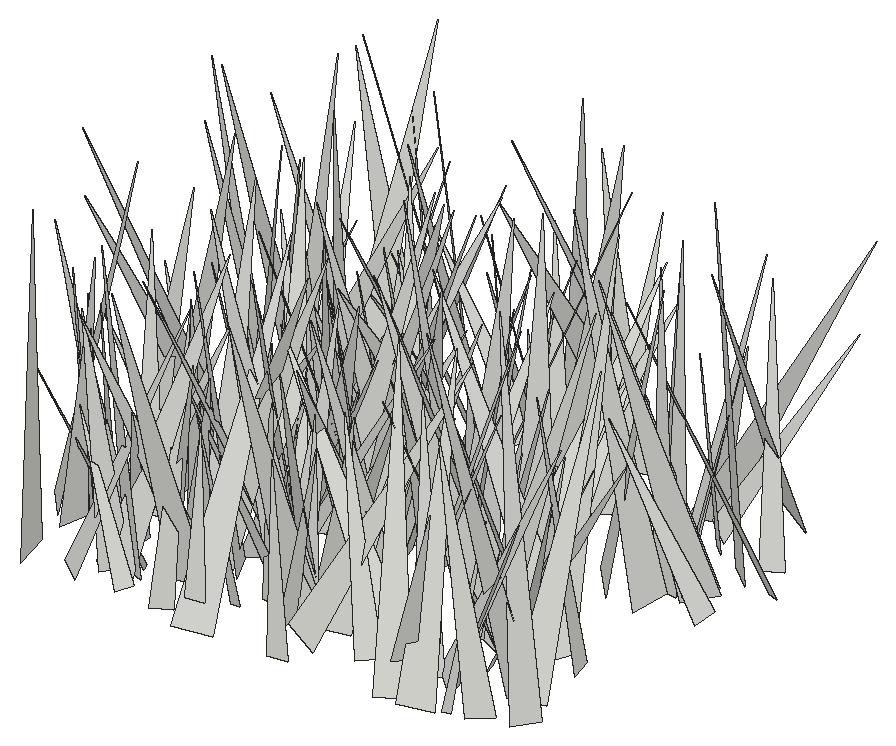
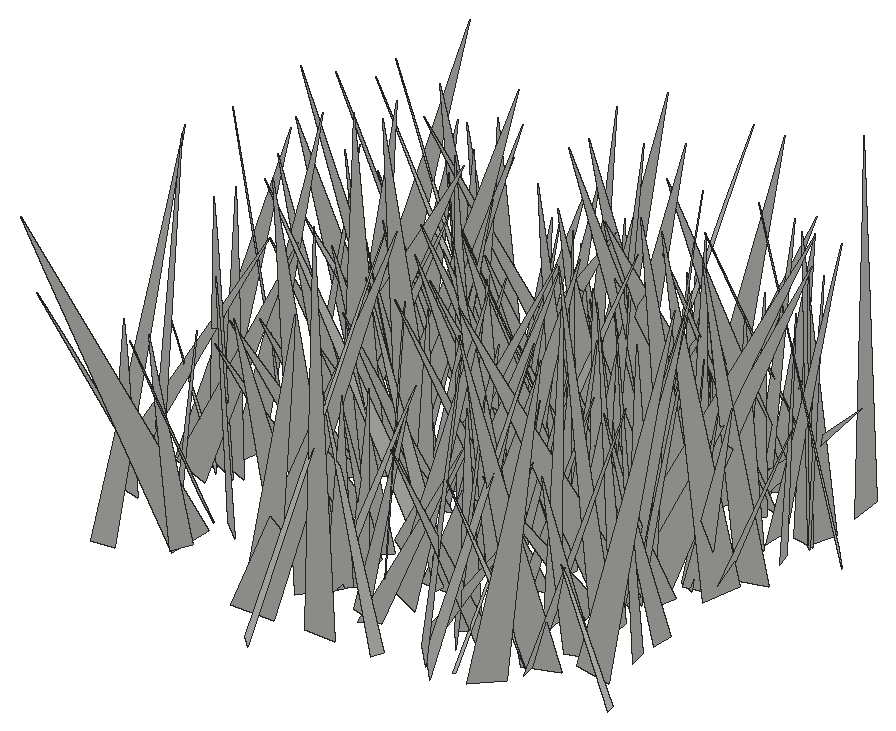
# SketchUp Ruby script. Lengths in inches.
U = 1.inch
M = Sketchup.active_model
def pt(a) = Geom::Point3d.new(a.map { |v| v * U })
def face(e, loops, mat)
  f = e.add_face(loops[0].map { |a| pt(a) })
  loops[1..].each { |l| e.add_face(l.map { |a| pt(a) }).erase! }
  f.material = f.back_material = mat if mat
  f
end
# faces: each face lists its corners as indices into pts; further lists are holes
def faces(e, pts, list, mat = nil) = list.each { |f| face(e, (f[0].is_a?(Array) ? f : [f]).map { |l| l.map { |i| pts[i] } }, mat) }
# xy, xz, yz: faces in a plane at the given z, y or x. An outline is a flat list of corners, or four numbers for a rectangle; further outlines are holes
def ring(l) = l.size == 4 ? [[l[0], l[1]], [l[2], l[1]], [l[2], l[3]], [l[0], l[3]]] : l.each_slice(2).to_a
def flat(e, list, mat, &to3) = list.each { |f| face(e, (f[0].is_a?(Array) ? f : [f]).map { |l| ring(l).map { |u, v| to3.(u, v) } }, mat) }
def xy(e, z, list, mat = nil) = flat(e, list, mat) { |x, y| [x, y, z] }
def xz(e, y, list, mat = nil) = flat(e, list, mat) { |x, z| [x, y, z] }
def yz(e, x, list, mat = nil) = flat(e, list, mat) { |y, z| [x, y, z] }
def lines(e, pts, list) = list.each { |a, b| e.add_line(pt(pts[a]), pt(pts[b])) }
# prism: a flat outline (further loops are holes) pulled along v
def prism(e, loops, v, mat = nil)
  f = face(e, loops, mat); d = Geom::Vector3d.new(v.map { |x| x * U })
  f.pushpull(f.normal.samedirection?(d) ? d.length : -d.length)
end
def box(e, o, s, mat = nil) = prism(e, [[o, [o[0] + s[0], o[1], o[2]], [o[0] + s[0], o[1] + s[1], o[2]], [o[0], o[1] + s[1], o[2]]]], [0, 0, s[2]], mat)
def at(x, y, z, deg = 0) = Geom::Transformation.translation(pt([x, y, z])) * Geom::Transformation.rotation(ORIGIN, Z_AXIS, deg.degrees)
def axes(o, x, y, z) = Geom::Transformation.new([*x, 0, *y, 0, *z, 0, *pt(o).to_a, 1])
def part(name) = M.definitions.add(name)
# library, detail: a bought-in or finely detailed component or shape, given as its bounding box
def library(name, o, s) = part(name).tap { |d| box(d.entities, o, s) }
def detail(e, o, s) = box(e.add_group.entities, o, s)
def put(e, d, t, mat = nil) = e.add_instance(d, t).tap { |i| i.material = mat if mat }
def group(e, t, mat = nil) = e.add_group.tap { |g| g.transformation = t; g.material = mat if mat }.entities
root = M.entities
c1 = part("fur_instance\#9")
p = [[0.8125,0,1.79],[0.67,-0.02,1.48],[0,-0.11,0],[0,0.11,0]]
faces(c1.entities,p,[[0,1,2,3]])
put(root,c1,axes([494.97,21.67,-21.86],[-0.42877,3.87256,1.55947],[4.17346,0.35848,0.25729],[-0.1042,-1.57711,3.88772]))
put(root,c1,axes([482.625,22.34,-21.86],[7.19679,1.10507,2.93039],[1.40985,-7.70082,-0.55845],[-2.79655,-1.03845,7.25969]))
put(root,c1,axes([499.85,22.83,-21.86],[2.67886,-4.09104,0.57639],[-4.11516,-2.58128,0.80469],[0.36641,0.91951,4.82342]))
put(root,c1,axes([490.95,21.67,-21.86],[-3.06481,2.41196,1.362],[2.48233,3.29293,-0.24563],[1.22908,-0.63618,3.89234]))
put(root,c1,axes([488.76,24.21,-21.86],[1.44091,-6.85532,1.40735],[-6.89305,-1.6385,-0.92385],[-1.20912,1.1714,6.94393]))
put(root,c1,axes([487.16,22.27,-21.86],[-3.33504,1.53851,0.16438],[1.54705,3.32218,0.29368],[0.02564,-0.33558,3.66104]))
put(root,c1,axes([485.94,23.24,-21.86],[3.52477,-3.78027,2.43443],[-3.94318,-4.08529,-0.63451],[-2.1606,1.28874,5.1295]))
put(root,c1,axes([493.65,24.95,-21.86],[2.47706,-6.70826,1.39737],[-6.69174,-2.68793,-1.04158],[-1.47445,0.92925,7.07472]))
put(root,c1,axes([503.74,22.87,-21.86],[-2.10663,5.00928,1.58804],[5.23429,1.84857,1.1125],[-0.46582,-1.88217,5.31913]))
put(root,c1,axes([488.68,25.03,-21.86],[1.14957,-5.99203,1.40359],[-5.68779,-1.57972,-2.08556],[-2.35023,0.89221,5.73379]))
put(root,c1,axes([484.65,22.14,-21.86],[3.5807,5.01538,0.32607],[5.01642,-3.54168,-0.61141],[0.30977,-0.61982,6.13202]))
put(root,c1,axes([493.22,25.93,-21.86],[-2.08812,-6.42397,1.05341],[-6.15561,2.30841,1.87538],[2.11792,0.37569,6.48927]))
put(root,c1,axes([501.36,21.95,-21.86],[-1.91608,6.79372,1.10059],[6.8739,1.94553,-0.04218],[0.33984,-1.04766,7.05863]))
put(root,c1,axes([500.21,22.02,-21.86],[-2.69969,6.39263,0.77147],[6.43614,2.65406,0.5304],[-0.19237,-0.91623,6.91901]))
put(root,c1,axes([485.48,25.29,-21.86],[4.01305,-1.4697,0.35123],[-1.33059,-3.90931,-1.15533],[-0.71618,-0.97223,4.11458]))
put(root,c1,axes([486.75,23.35,-21.86],[-3.5063,-5.04513,2.56803],[-5.65565,3.25438,-1.32851],[0.24851,2.88062,5.99854]))
put(root,c1,axes([493.62,23.95,-21.86],[3.83893,-0.81047,1.08867],[-0.8917,-3.9684,0.19003],[-1.0232,0.41758,3.91895]))
put(root,c1,axes([501.65,23.85,-21.86],[4.10602,0.97464,0.35289],[0.9844,-4.11806,-0.08026],[-0.32469,-0.15985,4.21935]))
put(root,c1,axes([504.2,24.85,-21.86],[-1.47229,-7.46087,2.3597],[-7.72207,0.99683,-1.66627],[-1.2659,2.59656,7.41996]))
put(root,c1,axes([491.17,23.9,-21.86],[0.98464,3.25356,1.70885],[3.23357,-1.6077,1.19779],[-1.74639,-1.14237,3.18127]))
put(root,c1,axes([498.42,24.57,-21.86],[5.98331,3.57339,0.75673],[3.63565,-5.68637,-1.89446],[0.35186,-2.00943,6.70672]))
put(root,c1,axes([502.5,22.4,-21.86],[1.53322,3.39,0.04746],[3.12816,-1.43461,1.41479],[-1.30727,0.54307,3.44111]))
put(root,c1,axes([489.17,21.97,-21.86],[-5.33411,1.7362,0.45715],[1.45522,5.02033,-2.08679],[1.05153,1.85957,5.20696]))
put(root,c1,axes([501.01,24.16,-21.86],[3.86219,5.07234,0.99731],[5.04282,-3.42294,-2.11973],[1.1372,-2.04809,6.01264]))
put(root,c1,axes([497.7,23.73,-21.86],[-2.79772,3.91125,0.86225],[4.00509,2.73873,0.57209],[0.02536,-1.03446,4.77471]))
put(root,c1,axes([486,23.1,-21.86],[-0.17372,7.00266,1.70424],[6.95108,0.61311,-1.81067],[1.90374,-1.5996,6.76675]))
put(root,c1,axes([486.73,24.05,-21.86],[-3.03964,-3.22245,0.08473],[-2.53096,2.3136,-2.80576],[-1.9964,1.97328,3.42802]))
put(root,c1,axes([482.43,25.15,-21.86],[5.9168,-1.45412,1.7202],[-1.44139,-6.15974,-0.24915],[-1.73089,0.15879,6.08776]))
put(root,c1,axes([486.95,25.27,-21.86],[4.77554,-0.30271,1.03368],[-0.19329,-4.86277,-0.53104],[-1.0596,-0.47722,4.75556]))
put(root,c1,axes([500.22,24.13,-21.86],[2.13883,-4.28297,3.06723],[-5.00629,-2.68295,-0.2554],[-1.63976,2.60467,4.7805]))
put(root,c1,axes([500.2,24.65,-21.86],[3.13012,3.09581,1.75638],[3.35561,-3.34662,-0.08138],[-1.18695,-1.29717,4.40172]))
put(root,c1,axes([489.71,28.34,-21.86],[-5.6893,-5.57398,0.54513],[-5.22917,5.56506,2.3282],[2.00554,-1.30211,7.61688]))
put(root,c1,axes([494.68,23.44,-21.86],[1.86343,6.88556,0.79652],[6.51007,-1.45535,-2.64927],[2.37997,-1.41024,6.62304]))
put(root,c1,axes([482.91,25.7,-21.86],[-1.22041,-5.00142,1.71972],[-5.19067,1.47111,0.5948],[1.01418,1.51086,5.11369]))
put(root,c1,axes([494.08,24.625,-21.86],[3.56835,-1.26097,2.05366],[-1.59686,-3.9854,0.32755],[-1.80488,1.03305,3.77039]))
put(root,c1,axes([482.85,25.64,-21.86],[-3.25997,-4.21096,1.97124],[-4.4396,3.53441,0.20814],[1.38129,1.42168,5.3213]))
put(root,c1,axes([491.15,21.32,-21.86],[-6.13074,4.86156,0.06985],[4.48302,5.69573,-2.94734],[1.88206,2.26926,7.24803]))
put(root,c1,axes([492.27,25.45,-21.86],[-2.15609,-3.98258,0.83043],[-3.73233,1.56246,-2.1972],[-1.61872,1.70208,3.96005]))
put(root,c1,axes([485.39,24.54,-21.86],[2.79379,4.96818,0.70977],[4.95175,-2.59669,-1.31495],[0.8165,-1.25148,5.54607]))
put(root,c1,axes([483.9,26.1,-21.86],[-6.39617,-0.72322,1.67284],[-0.5993,6.59982,0.56183],[1.72113,-0.38959,6.41236]))
put(root,c1,axes([499.16,23.59,-21.86],[5.77926,4.78065,0.80242],[4.74367,-5.8345,0.5954],[-0.99801,-0.04845,7.47663]))
put(root,c1,axes([487.12,26.49,-21.86],[3.8804,-2.67072,0.47699],[-2.66948,-3.90717,-0.15997],[-0.48385,0.13783,4.70793]))
put(root,c1,axes([489.6,26.19,-21.86],[-5.57513,-2.9786,1.92177],[-3.03694,5.86084,0.2736],[1.82819,0.65252,6.315]))
put(root,c1,axes([498.49,24.61,-21.86],[-3.37764,5.82202,0.02709],[5.22944,3.02002,2.9728],[-2.55923,-1.51283,6.03878]))
put(root,c1,axes([505.35,23.58,-21.86],[-7.7657,1.30292,0.44128],[1.14319,7.51969,-2.08465],[0.76515,1.98873,7.59328]))
put(root,c1,axes([491.97,24.86,-21.86],[1.9045,4.44389,1.45881],[4.34306,-2.26488,1.22946],[-1.73613,-0.79091,4.67587]))
put(root,c1,axes([495.52,24.64,-21.86],[-2.78361,3.37072,1.19614],[3.02117,3.0272,-1.49988],[1.91443,0.12385,4.10617]))
put(root,c1,axes([486.87,27.04,-21.86],[-1.17903,-5.46423,1.73554],[-5.62366,1.44698,0.7353],[1.11548,1.51937,5.54141]))
put(root,c1,axes([500.27,27.97,-21.86],[-4.1053,-4.23157,0.31859],[-4.21802,4.11764,0.33835],[0.46467,-0.00766,5.88602]))
put(root,c1,axes([482.67,27.21,-21.86],[4.23333,1.58778,2.03705],[2.11026,-4.38143,-0.97034],[-1.48911,-1.69519,4.41595]))
put(root,c1,axes([491.32,26.9,-21.86],[1.07794,-7.21694,3.00432],[-7.53412,-1.768,-1.54384],[-2.08502,2.65746,7.13181]))
put(root,c1,axes([501.82,27.74,-21.86],[4.97063,-0.22915,0.23226],[-0.15729,-4.7897,-1.3593],[-0.28585,-1.34904,4.78665]))
put(root,c1,axes([481.07,25.79,-21.86],[-4.56158,-4.36485,4.54967],[-5.17144,5.80258,0.38189],[3.60662,2.79958,6.30192]))
put(root,c1,axes([492.98,27.29,-21.86],[2.11868,-4.0714,0.72457],[-4.11944,-2.00647,0.77101],[0.3627,0.99394,4.52445]))
put(root,c1,axes([488.42,25.94,-21.86],[3.6811,-6.05089,2.6185],[-6.53456,-2.94932,2.37094],[0.87715,3.42178,6.67401]))
put(root,c1,axes([487.34,27.34,-21.86],[6.73019,-3.63445,0.24466],[-3.63894,-6.68481,0.79754],[0.16506,0.81773,7.60715]))
put(root,c1,axes([496.06,27.33,-21.86],[-0.12405,-5.8754,2.10648],[-6.00776,-0.4589,-1.63376],[-1.69244,2.05962,5.64504]))
put(root,c1,axes([492.49,25.67,-21.86],[-4.55508,3.55475,2.05706],[3.40532,4.98624,-1.07596],[2.29598,-0.34303,5.67691]))
put(root,c1,axes([489.74,29.15,-21.86],[-3.32814,-6.39102,1.50803],[-6.07577,3.63841,2.01068],[2.49085,0.3356,6.91945]))
put(root,c1,axes([492.43,30.06,-21.86],[5.08436,-3.96797,0.13679],[-3.71243,-4.83007,-2.12193],[-1.40762,-1.5937,6.0904]))
put(root,c1,axes([499.75,28.29,-21.86],[2.58278,-6.81445,2.81399],[-6.72051,-3.40212,-2.07037],[-3.03151,1.73634,6.98721]))
put(root,c1,axes([504.35,24.96,-21.86],[-4.09876,5.0884,1.14662],[4.86258,4.25523,-1.50159],[1.8873,0.0873,6.359]))
put(root,c1,axes([495.31,27.3,-21.86],[-3.89447,-3.70378,1.65585],[-4.00703,3.87088,-0.766],[0.63525,1.71028,5.3196]))
put(root,c1,axes([489.3,27.12,-21.86],[3.48145,-1.92251,0.90917],[-2.10367,-3.36896,0.93158],[-0.31179,1.26381,3.86636]))
put(root,c1,axes([501.71,25.92,-21.86],[4.18382,1.92252,0.07247],[1.86113,-4.08842,1.01327],[-0.48737,0.89131,4.49152]))
put(root,c1,axes([490.24,27.52,-21.86],[3.88099,1.49769,1.22771],[1.56049,-4.04689,0.00388],[-1.14683,-0.43823,4.15995]))
put(root,c1,axes([495.72,26.625,-21.86],[3.85077,0.95797,1.10657],[0.6489,-3.90916,1.12606],[-1.31192,0.87829,3.80501]))
put(root,c1,axes([504.36,28.1,-21.86],[-5.31437,-1.63311,1.48269],[-1.72892,5.48589,-0.1545],[1.36976,0.58821,5.55749]))
put(root,c1,axes([484.32,27.25,-21.86],[-1.52023,5.3398,1.43684],[5.52962,1.4775,0.35965],[0.03531,-1.48075,5.54032]))
put(root,c1,axes([501.79,28.69,-21.86],[-3.22494,-3.97651,0.65226],[-4.0077,3.07801,-1.05003],[-0.42001,1.16258,5.01102]))
put(root,c1,axes([502.84,26.62,-21.86],[-3.9364,0.91485,1.26316],[0.41585,3.92071,-1.54367],[1.50319,1.31107,3.73488]))
put(root,c1,axes([495.43,30.68,-21.86],[5.19652,-2.78136,0.42044],[-2.54268,-5.02221,-1.79688],[-1.20313,-1.39929,5.61347]))
put(root,c1,axes([484.32,29.1875,-21.86],[3.64013,-0.49009,0.65042],[-0.33955,-3.62113,-0.82821],[-0.74023,-0.74902,3.57838]))
put(root,c1,axes([500.47,27.47,-21.86],[2.40948,7.1196,1.80641],[7.28749,-2.07931,-1.52526],[0.91887,-2.17835,7.35989]))
put(root,c1,axes([485.63,29.3,-21.86],[-2.68709,-2.60275,1.28992],[-2.48203,2.97011,0.82256],[1.50922,0.25052,3.6494]))
put(root,c1,axes([487.46,27.38,-21.86],[-1.01475,7.09695,1.79918],[7.31311,1.06925,-0.09303],[0.3496,-1.76734,7.16853]))
put(root,c1,axes([500.15,27.84,-21.86],[-3.37958,0.77927,1.41196],[0.41341,3.58754,-0.99047],[1.55884,0.73803,3.32382]))
put(root,c1,axes([498,31.15,-21.86],[-3.1075,-6.9448,0.74353],[-6.98342,3.07514,-0.46373],[-0.12218,0.86773,7.5942]))
put(root,c1,axes([503.27,28.45,-21.86],[-3.57057,6.8988,1.02898],[6.50769,2.8788,3.28081],[-2.51043,-2.34953,7.04122]))
put(root,c1,axes([485.45,31.43,-21.86],[0.03934,-7.1777,0.79174],[-6.87762,-0.27857,-2.18369],[-2.20103,0.74216,6.83757]))
put(root,c1,axes([487.04,30.35,-21.86],[-3.02685,-7.70536,1.30124],[-7.48247,2.45538,-2.86554],[-2.25353,2.19686,7.76679]))
put(root,c1,axes([482.41,29.34,-21.86],[0.14436,6.2225,2.72909],[6.68972,0.34776,-1.14678],[1.18962,-2.71069,6.11762]))
put(root,c1,axes([489.3,31.47,-21.86],[1.41766,-6.83451,0.48866],[-6.53171,-1.19719,2.20513],[2.07029,0.90294,6.62252]))
put(root,c1,axes([490.17,29.31,-21.86],[4.83025,3.81866,0.07193],[3.65702,-4.5907,-1.86288],[1.10161,-1.50398,5.86882]))
put(root,c1,axes([483.11,30.47,-21.86],[-3.67924,-0.76157,0.35539],[-0.68587,3.64327,0.70657],[0.48566,-0.62424,3.6902]))
put(root,c1,axes([500.62,29.39,-21.86],[4.05513,-1.76427,0.28786],[-1.75227,-3.78191,1.50543],[0.35366,1.49134,4.15818]))
put(root,c1,axes([492.39,30.83,-21.86],[-4.77204,-4.71706,0.72174],[-4.75307,4.60775,-1.31181],[-0.42413,1.43592,6.58044]))
put(root,c1,axes([489.92,29.1875,-21.86],[4.13014,0.16234,0.60229],[0.00137,-4.03539,1.07832],[-0.62379,1.06603,3.99019]))
put(root,c1,axes([495.38,31.84,-21.86],[-1.39577,-4.42794,0.41329],[-4.44248,1.40819,0.08395],[0.20461,0.36877,4.64196]))
put(root,c1,axes([484.2,31.07,-21.86],[-1.43466,-3.23484,0.82707],[-3.31328,1.49057,0.08262],[0.41278,0.72144,3.53774]))
put(root,c1,axes([493.85,30.84,-21.86],[3.71055,0.76796,0.33165],[0.80764,-3.68168,-0.51076],[-0.21789,-0.56867,3.7546]))
put(root,c1,axes([489.46,31.23,-21.86],[3.61055,-0.61097,0.20103],[-0.59508,-3.6081,-0.27795],[-0.24409,-0.24103,3.65131]))
put(root,c1,axes([482.8,30.74,-21.86],[7.15421,-1.9799,2.12173],[-2.22149,-7.36827,0.61487],[-1.86728,1.18029,7.39761]))
put(root,c1,axes([491.57,31.54,-21.86],[-3.854,-0.48704,1.31581],[-0.33639,4.05498,0.51565],[1.36213,-0.37663,3.85028]))
put(root,c1,axes([485.37,32.37,-21.86],[3.21105,-3.45107,0.18225],[-3.45172,-3.21492,-0.06213],[-0.16965,0.09106,4.71348]))
put(root,c1,axes([497.25,29.95,-21.86],[4.98467,2.72403,1.68688],[2.57744,-5.26236,0.88159],[-1.90334,0.00786,5.61161]))
put(root,c1,axes([483.81,31.04,-21.86],[1.42744,-3.53628,2.17287],[-3.81125,-2.02664,-0.79456],[-1.64348,1.62839,3.72982]))
put(root,c1,axes([493.47,30.15,-21.86],[5.10289,-1.83511,1.25864],[-2.13691,-4.91957,1.49087],[-0.62081,1.84972,5.21387]))
put(root,c1,axes([484.53,32.9375,-21.86],[3.64505,-0.39812,0.27738],[-0.20845,-3.18305,-1.82936],[-0.43816,-1.79764,3.17779]))
put(root,c1,axes([491.24,30.07,-21.86],[-0.29614,5.30233,1.4786],[4.87042,0.94241,-2.40408],[2.56516,-1.17721,4.73528]))
put(root,c1,axes([498.14,30.67,-21.86],[4.26152,0.65659,1.09682],[0.47447,-4.35714,0.76482],[-1.18701,0.6156,4.24343]))
put(root,c1,axes([492.12,34.08,-21.86],[-0.39765,-7.51588,0.89638],[-7.02687,0.7002,2.75371],[2.81337,0.68655,7.00455]))
put(root,c1,axes([488.26,33.1,-21.86],[6.38697,0.74513,2.00431],[1.2691,-6.40204,-1.66407],[-1.72101,-1.95564,6.21124]))
put(root,c1,axes([496.31,31.16,-21.86],[-7.25051,-1.24633,1.39987],[-1.43303,7.2913,-0.93068],[1.20805,1.16894,7.29774]))
put(root,c1,axes([502.8,28.72,-21.86],[0.70826,8.01559,0.32411],[7.89046,-0.75477,1.42384],[-1.44754,-0.19233,7.91985]))
put(root,c1,axes([484.96,33.02,-21.86],[-2.78076,-3.999,1.01738],[-3.97731,2.92434,0.62365],[1.09912,0.46468,4.83071]))
put(root,c1,axes([492.08,29.42,-21.86],[7.02888,1.27959,1.54515],[0.73768,-6.88381,2.34499],[-1.86566,2.099,6.7486]))
put(root,c1,axes([496.07,32.11,-21.86],[-3.12669,6.25889,3.83958],[6.87271,3.96367,-0.86451],[2.58493,-2.9678,6.9428]))
put(root,c1,axes([484.08,32.61,-21.86],[2.63596,-3.80697,0.02165],[-3.40971,-2.34911,2.07299],[1.69332,1.196,4.14053]))
put(root,c1,axes([488.36,30.5,-21.86],[-3.98192,5.65644,1.02142],[5.69703,4.04883,-0.21229],[0.76316,-0.7113,6.91418]))
put(root,c1,axes([498.92,32.05,-21.86],[4.92232,-5.34816,3.43981],[-5.97476,-5.37881,0.1869],[-2.17654,2.67018,7.26616]))
put(root,c1,axes([490.71,30.38,-21.86],[6.0321,-2.57805,3.10449],[-3.62742,-5.91038,2.14001],[-1.76807,3.33038,6.20104]))
put(root,c1,axes([494.87,33.46,-21.86],[3.43508,-2.31671,0.74566],[-2.27877,-3.51457,-0.42176],[-0.85461,0.05948,4.12177]))
put(root,c1,axes([491.71,33.29,-21.86],[0.21483,-6.37799,2.26736],[-6.52313,-0.80094,-1.63496],[-1.80789,2.13204,6.16862]))
put(root,c1,axes([488.375,31.78,-21.86],[-2.8304,4.89567,0.80261],[4.94903,2.72215,0.8485],[-0.34477,-1.11592,5.59096]))
put(root,c1,axes([490.79,32.74,-21.86],[-3.38469,-3.26483,1.22467],[-3.48648,3.19729,-1.11215],[0.05857,1.65326,4.56929]))
put(root,c1,axes([490.5,31.24,-21.86],[6.56769,-0.93589,1.93904],[-1.50422,-6.44796,1.98276],[-1.54048,2.30611,6.3308]))
put(root,c1,axes([505.54,34.06,-21.86],[-4.40105,0.97982,0.44244],[1.06612,4.21791,1.26401],[0.13855,-1.33202,4.328]))
put(root,c1,axes([488.54,33.08,-21.86],[-5.34365,-1.01248,1.41227],[-1.15776,5.47992,-0.452],[1.29585,0.72082,5.4199]))
put(root,c1,axes([500.875,33.84,-21.86],[5.37674,4.78999,2.15375],[5.23773,-5.117,-1.69543],[-0.38579,-2.71372,6.99849]))
put(root,c1,axes([504.49,35.11,-21.86],[3.31279,-6.01066,2.01721],[-5.81791,-3.7865,-1.72802],[-2.51972,0.84034,6.64203]))
put(root,c1,axes([485.45,34.19,-21.86],[-1.73003,-6.76572,2.01517],[-7.01807,1.42401,-1.24409],[-0.76325,2.2419,6.8717]))
put(root,c1,axes([493.37,31.55,-21.86],[-5.19034,4.80556,0.45379],[4.78626,5.21014,-0.43029],[0.62529,0.00866,7.0603]))
put(root,c1,axes([503.22,33.68,-21.86],[-8.03417,0.61584,1.78735],[0.70083,8.21761,0.3188],[1.75577,-0.4621,8.05143]))
put(root,c1,axes([491.41,37.01,-21.86],[4.98513,-4.06782,0.78587],[-3.3159,-4.65458,-3.05875],[-2.48386,-1.95039,5.66063]))
put(root,c1,axes([495.39,33.05,-21.86],[-3.61899,-3.55384,3.43713],[-4.24844,4.41399,0.09065],[2.52873,2.32973,5.07136]))
put(root,c1,axes([494.15,35.65,-21.86],[-3.14306,-6.22127,0.26286],[-6.12359,3.03481,-1.39417],[-1.12913,0.859,6.8293]))
put(root,c1,axes([486.93,35.35,-21.86],[4.79188,-1.27621,1.00499],[-1.01396,-4.79557,-1.25507],[-1.26909,-0.98723,4.79746]))
put(root,c1,axes([499.5625,32.17,-21.86],[-1.55041,4.4226,0.08121],[4.26043,1.51619,-1.23272],[1.18941,0.33394,4.52145]))
put(root,c1,axes([485.72,33.13,-21.86],[1.68916,7.29229,2.94864],[7.0223,-2.75681,2.79508],[-3.5439,-1.98689,6.94394]))
put(root,c1,axes([495.06,32.32,-21.86],[-0.26942,5.43204,0.24352],[5.36362,0.30555,-0.88154],[0.89325,-0.19629,5.36679]))
put(root,c1,axes([488.23,35.98,-21.86],[-4.24869,-0.73201,1.00331],[-0.4187,4.21079,1.29914],[1.16925,-1.15205,4.11089]))
put(root,c1,axes([484.12,35.27,-21.86],[6.17707,1.48648,1.9777],[1.80034,-6.34915,-0.85095],[-1.69697,-1.32504,6.29616]))
put(root,c1,axes([482.33,34.9,-21.86],[4.64255,0.07182,0.51653],[0.0806,-4.67045,-0.07504],[-0.51523,-0.08349,4.6425]))
put(root,c1,axes([491.99,35.26,-21.86],[-3.61147,3.35043,1.62323],[3.67501,3.56996,0.80783],[0.59541,-1.71259,4.85958]))
put(root,c1,axes([503.07,34.74,-21.86],[1.52535,6.05061,2.3847],[6.37233,-1.8801,0.69429],[-1.30004,-2.1163,6.20117]))
put(root,c1,axes([482.21,36.51,-21.86],[6.17791,2.14602,1.95241],[2.61385,-6.11017,-1.55482],[-1.25898,-2.15507,6.35252]))
put(root,c1,axes([488.74,36.18,-21.86],[-3.36264,-2.39418,1.21792],[-2.41208,3.55006,0.31902],[1.18208,0.43333,4.11555]))
put(root,c1,axes([494.43,34.11,-21.86],[7.40183,3.33475,0.3809],[3.31775,-7.40888,0.39208],[-0.5081,0.20159,8.10888]))
put(root,c1,axes([494.65,36.26,-21.86],[1.94389,-4.04886,0.80465],[-4.08173,-1.75236,1.04312],[0.61659,1.16421,4.36851]))
put(root,c1,axes([504.25,35.75,-21.86],[-0.7555,-5.85213,2.53673],[-5.87032,-0.36099,-2.58111],[-2.49433,2.62211,5.30623]))
put(root,c1,axes([503.69,34.95,-21.86],[2.95559,2.2846,0.71516],[2.24296,-3.03986,0.44126],[-0.83663,-0.07885,3.70947]))
put(root,c1,axes([485.125,33.8,-21.86],[6.18283,-3.26103,2.17206],[-3.91127,-5.37775,3.05962],[-0.2327,3.74499,6.28493]))
put(root,c1,axes([487.09,37.8,-21.86],[3.43044,-6.71204,0.2285],[-6.5076,-3.25868,1.97581],[1.6598,1.09595,7.27431]))
put(root,c1,axes([491.28,36.83,-21.86],[6.07626,0.90493,0.17774],[0.92213,-5.94508,-1.25588],[0.01299,-1.26833,6.01354]))
put(root,c1,axes([490.64,35.9,-21.86],[-2.6227,-3.62693,1.52989],[-3.9333,2.34177,-1.19122],[-0.15598,1.93268,4.31442]))
put(root,c1,axes([484.91,35.26,-21.86],[2.51079,7.35519,2.45383],[7.71335,-2.63218,-0.00261],[-0.79014,-2.32314,7.77193]))
put(root,c1,axes([488.22,34.76,-21.86],[1.82211,6.46965,0.85286],[6.26515,-1.48669,-2.10749],[1.8253,-1.35544,6.38239]))
put(root,c1,axes([503.49,34.87,-21.86],[1.52535,6.57132,1.88983],[6.63248,-1.89273,1.22809],[-1.66251,-1.52175,6.63331]))
put(root,c1,axes([486.22,36.6,-21.86],[-6.46976,-1.55499,2.98827],[-1.52534,7.12153,0.40334],[3.00351,0.26714,6.64177]))
put(root,c1,axes([506.49,36.96,-21.86],[-3.99389,-5.07881,0.29207],[-4.86869,3.70838,-2.09153],[-1.47493,1.51142,6.11318]))
put(root,c1,axes([485.8,34.74,-21.86],[3.8069,0.05751,0.20355],[-0.0416,-3.39391,1.73693],[-0.20739,1.73647,3.38805]))
put(root,c1,axes([493.69,37.28,-21.86],[-4.27511,-3.26782,2.05551],[-3.38668,4.64678,0.34365],[1.85313,0.95347,5.37002]))
put(root,c1,axes([482.75,38.52,-21.86],[-1.04582,-7.4675,1.55674],[-7.62212,0.96116,-0.50998],[-0.30029,1.61039,7.52311]))
put(root,c1,axes([497.15,34.57,-21.86],[-2.16647,5.60636,0.16983],[5.26617,2.09582,-2.00715],[1.93067,0.57445,5.66535]))
put(root,c1,axes([504.57,37.42,-21.86],[-4.94486,-5.49387,2.91837],[-6.02867,5.15162,-0.51692],[1.53451,2.53562,7.37341]))
put(root,c1,axes([488.39,38.77,-21.86],[1.68114,-3.92704,0.2758],[-3.91607,-1.63754,0.5539],[0.40264,0.46985,4.23569]))
put(root,c1,axes([491.82,38.52,-21.86],[-2.51805,-6.35566,1.6356],[-6.55451,2.34778,-0.96776],[-0.32873,1.87181,6.76746]))
put(root,c1,axes([493.81,38.75,-21.86],[3.2467,-2.02133,0.75684],[-1.94033,-3.33216,-0.57574],[-0.94537,-0.10279,3.78092]))
put(root,c1,axes([494.26,37.16,-21.86],[3.63401,0.67625,1.41653],[0.37628,-3.84346,0.86953],[-1.5239,0.6636,3.59267]))
put(root,c1,axes([496.37,36.3125,-21.86],[-1.05033,5.0969,0.69056],[4.61293,1.24522,-2.17458],[2.27512,-0.17172,4.72788]))
put(root,c1,axes([502.66,38.51,-21.86],[-2.70575,-2.79772,1.42447],[-3.05403,2.78134,-0.3384],[0.7275,1.27058,3.87735]))
put(root,c1,axes([503.31,42.18,-21.86],[-2.73458,-7.67612,0.26637],[-7.34259,2.69559,2.30041],[2.25392,-0.53168,7.81722]))
put(root,c1,axes([500.21,38.34,-21.86],[3.30572,4.13092,2.03155],[4.38871,-3.58299,0.14433],[-1.38957,-1.489,5.28881]))
put(root,c1,axes([494.85,38.65,-21.86],[-4.27144,-3.27285,0.83505],[-3.36103,3.98484,-1.57435],[-0.33515,1.75031,5.14569]))
put(root,c1,axes([484.89,39.49,-21.86],[-6.22564,-1.43503,0.72375],[-1.44178,6.26598,0.02194],[0.71021,0.14105,6.38885]))
put(root,c1,axes([495.66,42.79,-21.86],[3.75973,-6.87339,0.18092],[-6.4988,-3.61971,-2.46477],[-2.2454,-1.03249,7.43666]))
put(root,c1,axes([486.9,41.62,-21.86],[-2.93741,-3.09466,0.01129],[-2.71699,2.58635,2.03327],[1.48156,-1.39259,3.75115]))
put(root,c1,axes([492.45,40.32,-21.86],[-1.40933,-4.17013,0.64925],[-4.20295,1.44894,0.18319],[0.38311,0.55526,4.39803]))
put(root,c1,axes([494.73,39.95,-21.86],[5.49312,-5.94068,1.74056],[-6.16398,-5.4638,0.80479],[-0.57141,1.8305,8.05098]))
put(root,c1,axes([497.69,37.98,-21.86],[-4.4871,3.83069,1.41429],[3.5666,4.69982,-1.41404],[1.98841,0.2144,5.72789]))
put(root,c1,axes([484.03,37.73,-21.86],[-1.75814,5.2069,0.13379],[5.20853,1.75836,0.01288],[0.0306,-0.13088,5.4957]))
put(root,c1,axes([480.6,40.16,-21.86],[3.77978,1.93812,0.15141],[1.88384,-3.56988,-1.33157],[0.48001,-1.25124,4.0336]))
put(root,c1,axes([491.79,40.61,-21.86],[-4.14397,2.00475,0.46664],[2.04964,3.92263,1.34951],[-0.1891,-1.41534,4.40117]))
put(root,c1,axes([494.22,39.39,-21.86],[-4.07522,2.66076,1.05763],[2.66001,4.19896,-0.31421],[1.05952,-0.30776,4.85678]))
put(root,c1,axes([500.86,40.53,-21.86],[3.79566,-1.87078,0.73995],[-1.92959,-3.83243,0.2087],[-0.56925,0.51676,4.2265]))
put(root,c1,axes([488.54,39.51,-21.86],[3.70498,4.05955,2.96614],[3.93602,-4.63444,1.42637],[-3.1282,-1.02317,5.30776]))
put(root,c1,axes([505.26,38.43,-21.86],[-0.43332,5.55714,0.38235],[5.39105,0.32188,1.43136],[-1.40165,-0.47995,5.3871]))
put(root,c1,axes([489.26,40.22,-21.86],[-2.6027,-3.00196,0.39616],[-2.70686,2.07255,-2.07851],[-1.35707,1.62343,3.38609]))
put(root,c1,axes([501.88,37.73,-21.86],[2.78013,5.13783,0.11647],[4.85085,-2.66723,1.86951],[-1.69707,0.79284,5.53456]))
put(root,c1,axes([501.78,39.57,-21.86],[2.70061,4.81345,0.08968],[4.52857,-2.505,-1.92033],[1.63383,-1.01307,5.17446]))
put(root,c1,axes([488.58,41.36,-21.86],[-4.69837,-4.55111,2.1601],[-4.81656,4.92378,-0.10244],[1.47629,1.58022,6.5404]))
put(root,c1,axes([484.49,39.43,-21.86],[-1.03239,7.59334,1.92082],[7.72051,1.31303,-1.04105],[1.31985,-1.74108,7.59215]))
put(root,c1,axes([485.52,41.43,-21.86],[-5.98098,3.27291,2.42019],[3.72115,6.13978,0.89298],[1.64993,-1.98304,6.75918]))
put(root,c1,axes([487.02,39.46,-21.86],[4.77629,1.47467,0.59608],[1.29577,-4.70156,1.24867],[-0.92247,1.03128,4.84029]))
put(root,c1,axes([485.45,39.19,-21.86],[3.76197,3.17485,0.58422],[2.97684,-3.75885,1.25811],[-1.24876,0.60394,4.75913]))
put(root,c1,axes([494.48,44.64,-21.86],[-6.0329,-5.73941,0.68236],[-5.34499,5.91535,2.49841],[2.19943,-1.36753,7.94322]))
put(root,c1,axes([490.02,42.36,-21.86],[5.19096,1.17327,0.15724],[1.14991,-4.82989,-1.92283],[0.28108,-1.90867,4.96239]))
put(root,c1,axes([488.01,41.84,-21.86],[-5.67662,-5.13617,1.32256],[-5.29359,5.60645,-0.94818],[0.32758,1.59402,7.59639]))
put(root,c1,axes([500.88,39.97,-21.86],[6.56364,-3.25708,1.01889],[-3.38805,-5.95385,2.79299],[0.40967,2.94467,6.77415]))
put(root,c1,axes([492.59,42.57,-21.86],[-1.23371,-7.71978,2.49826],[-7.92295,1.69122,1.31342],[1.75022,2.21429,7.70662]))
put(root,c1,axes([496.52,41.125,-21.86],[-1.23354,6.12021,2.2306],[6.48252,0.93032,1.03231],[-0.63996,-2.37312,6.15735]))
